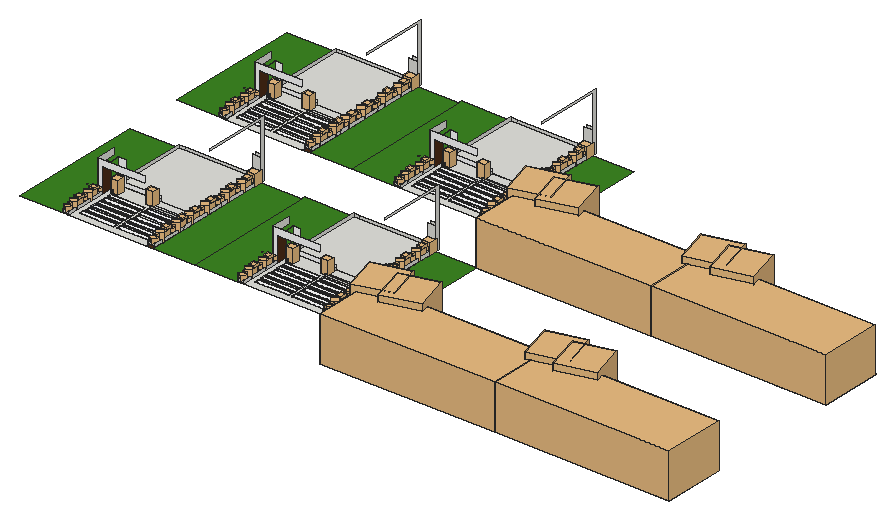
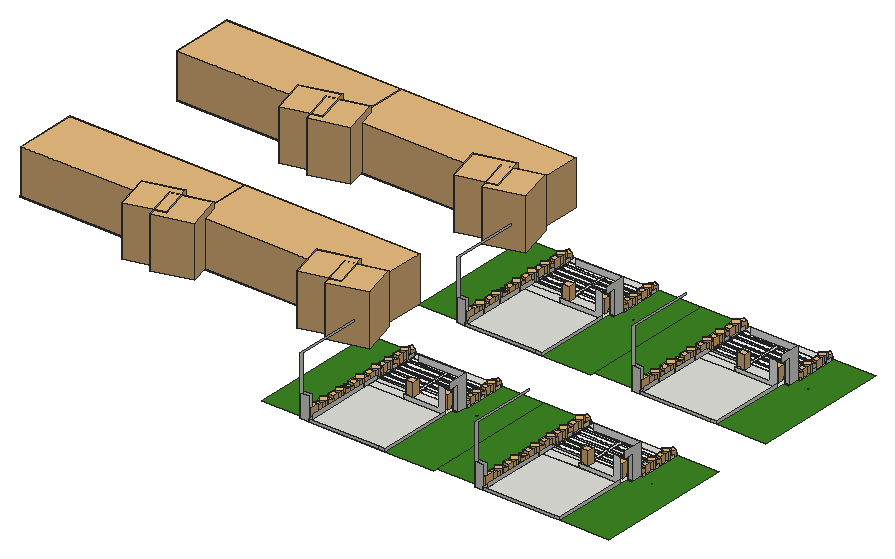
# SketchUp Ruby script. Lengths in inches.
U = 1.inch
M = Sketchup.active_model
def pt(a) = Geom::Point3d.new(a.map { |v| v * U })
def face(e, loops, mat)
  f = e.add_face(loops[0].map { |a| pt(a) })
  loops[1..].each { |l| e.add_face(l.map { |a| pt(a) }).erase! }
  f.material = f.back_material = mat if mat
  f
end
# faces: each face lists its corners as indices into pts; further lists are holes
def faces(e, pts, list, mat = nil) = list.each { |f| face(e, (f[0].is_a?(Array) ? f : [f]).map { |l| l.map { |i| pts[i] } }, mat) }
# xy, xz, yz: faces in a plane at the given z, y or x. An outline is a flat list of corners, or four numbers for a rectangle; further outlines are holes
def ring(l) = l.size == 4 ? [[l[0], l[1]], [l[2], l[1]], [l[2], l[3]], [l[0], l[3]]] : l.each_slice(2).to_a
def flat(e, list, mat, &to3) = list.each { |f| face(e, (f[0].is_a?(Array) ? f : [f]).map { |l| ring(l).map { |u, v| to3.(u, v) } }, mat) }
def xy(e, z, list, mat = nil) = flat(e, list, mat) { |x, y| [x, y, z] }
def xz(e, y, list, mat = nil) = flat(e, list, mat) { |x, z| [x, y, z] }
def yz(e, x, list, mat = nil) = flat(e, list, mat) { |y, z| [x, y, z] }
def lines(e, pts, list) = list.each { |a, b| e.add_line(pt(pts[a]), pt(pts[b])) }
# prism: a flat outline (further loops are holes) pulled along v
def prism(e, loops, v, mat = nil)
  f = face(e, loops, mat); d = Geom::Vector3d.new(v.map { |x| x * U })
  f.pushpull(f.normal.samedirection?(d) ? d.length : -d.length)
end
def box(e, o, s, mat = nil) = prism(e, [[o, [o[0] + s[0], o[1], o[2]], [o[0] + s[0], o[1] + s[1], o[2]], [o[0], o[1] + s[1], o[2]]]], [0, 0, s[2]], mat)
def at(x, y, z, deg = 0) = Geom::Transformation.translation(pt([x, y, z])) * Geom::Transformation.rotation(ORIGIN, Z_AXIS, deg.degrees)
def axes(o, x, y, z) = Geom::Transformation.new([*x, 0, *y, 0, *z, 0, *pt(o).to_a, 1])
def part(name) = M.definitions.add(name)
# library, detail: a bought-in or finely detailed component or shape, given as its bounding box
def library(name, o, s) = part(name).tap { |d| box(d.entities, o, s) }
def detail(e, o, s) = box(e.add_group.entities, o, s)
def put(e, d, t, mat = nil) = e.add_instance(d, t).tap { |i| i.material = mat if mat }
def group(e, t, mat = nil) = e.add_group.tap { |g| g.transformation = t; g.material = mat if mat }.entities
root = M.entities
M.materials.add("Material__1").color = [95, 70, 46]
M.materials.add("[Carrera Marble]").color = [255, 255, 255]
M.materials.add("[Color M00]").color = [255, 255, 255]
M.materials.add("[Color M04]").color = [60, 133, 34]
M.materials.add("[Wood Veneer 01]").color = [76, 44, 23]
c1 = library("plant (1)",[-35.72,-28.42,0],[66.31,67.39,84.38])
c2 = library("Areca palm plant",[0,0,0],[49.1,36.6,54.46])
c3 = library("Group\#14",[-84.69,-90.07,-0.36],[176.51,175.13,171.4])
c4 = library("Group20\#1",[-20.81,-17.08,3.79],[39.86,39.43,37.51])
c5 = library("Group\#130",[-7.34,-1.2,0],[38.67,35.81,49.04])
c6 = library("Group38\#2",[14.01,28.44,-23.43],[18.58,18.32,38.89])
c7 = part("Group\#15")
xy(c7.entities,0,[[0,0,6,234.8],[30,0,36,234.8]])
xy(c7.entities,3,[[6,0,30,234.8]])
xy(c7.entities,7,[[6,5,30,229.8]],"Material__1")
xy(c7.entities,15,[[[0,0,36,234.8],[6,5,30,229.8]]])
xz(c7.entities,0,[[0,0,6,0,6,3,30,3,30,0,36,0,36,15,0,15]])
xz(c7.entities,5,[[6,7,30,15]])
xz(c7.entities,229.8,[[6,7,30,15]])
xz(c7.entities,234.8,[[0,0,0,15,36,15,36,0,30,0,30,3,6,3,6,0]])
yz(c7.entities,0,[[0,0,234.8,15]])
yz(c7.entities,6,[[0,0,234.8,3],[5,7,229.8,15]])
yz(c7.entities,30,[[0,0,234.8,3],[5,7,229.8,15]])
yz(c7.entities,36,[[0,0,234.8,15]])
c8 = part("Group\#17")
put(c8.entities,c2,axes([-6.2,56.6,6.08],[0.45017,-0.56191,0],[0.66137,0.52986,0],[0,0,0.72]))
put(c8.entities,c2,axes([-6.2,158.41,6.08],[0.45017,-0.56191,0],[0.66137,0.52986,0],[0,0,0.72]))
put(c8.entities,c3,axes([14.93,44.05,6.05],[-0.04961,-0.08593,0],[0.08593,-0.04961,0],[0,0,0.10522]))
put(c8.entities,c3,axes([14.93,71.3,6.05],[-0.04961,-0.08593,0],[0.08593,-0.04961,0],[0,0,0.10522]))
put(c8.entities,c4,axes([18.97,79.98,4.77],[0,0.85,0],[-0.85,0,0],[0,0,0.85]))
put(c8.entities,c3,axes([14.93,145.87,6.05],[-0.04961,-0.08593,0],[0.08593,-0.04961,0],[0,0,0.10522]))
put(c8.entities,c3,axes([17.19,15.79,6.07],[-0.08133,-0.14087,0],[0.14087,-0.08133,0],[0,0,0.1725]))
put(c8.entities,c3,axes([17.19,223.04,6.07],[-0.08133,-0.14087,0],[0.14087,-0.08133,0],[0,0,0.1725]))
put(c8.entities,c3,axes([17.19,121.23,6.07],[-0.08133,-0.14087,0],[0.14087,-0.08133,0],[0,0,0.1725]))
put(c8.entities,c5,axes([24.9375,191.72,8],[0,0.79,0],[-0.79,0,0],[0,0,0.79]))
put(c8.entities,c5,axes([24.9375,89.91,8],[0,0.79,0],[-0.79,0,0],[0,0,0.79]))
put(c8.entities,c3,axes([14.93,91.37,6.05],[-0.04961,-0.08593,0],[0.08593,-0.04961,0],[0,0,0.10522]))
put(c8.entities,c4,axes([18.97,181.79,4.77],[0,0.85,0],[-0.85,0,0],[0,0,0.85]))
put(c8.entities,c6,axes([-4.1,-1.15,28.17],[0.8848,0,0],[0,0.94674,0],[0,0,0.85826]))
put(c8.entities,c6,axes([-4.1,100.66,28.17],[0.8848,0,0],[0,0.94674,0],[0,0,0.85826]))
put(c8.entities,c7,at(0,0,0))
put(c8.entities,c3,axes([14.93,173.12,6.05],[-0.04961,-0.08593,0],[0.08593,-0.04961,0],[0,0,0.10522]))
put(c8.entities,c3,axes([14.93,193.18,6.05],[-0.04961,-0.08593,0],[0.08593,-0.04961,0],[0,0,0.10522]))
c9 = library("Plant",[0,0,0],[12.59,12.59,14.16])
c10 = library("plant1",[-367.84,-375.82,-125.45],[750.59,696.16,1346.74])
c11 = part("skp4FF")
put(c11.entities,c10,at(0,0,0))
c12 = library("BPJ-Road5D",[0,0,1],[442,720,229.125])
c13 = library("Palm tree",[-4.09,-4.52,0],[193.52,193.51,258.93])
c14 = part("Palm+Tree")
put(c14.entities,c13,at(25.51,-21.81,0,15))
xy(root,-19.54,[[[279.74,317.81,671.36,317.81,671.36,570.37,491.71,570.37,491.71,638.99,279.74,638.99,279.74,595.43,252.74,595.43,252.74,588.74,279.74,588.74],[493.96,534.6,667.46,556.1],[493.96,464.47,667.46,485.97],[493.96,429.41,667.46,450.91],[493.96,394.35,667.46,415.85],[493.96,359.29,667.46,380.79],[305.46,534.6,478.96,556.1],[305.46,464.47,478.96,485.97],[305.46,429.41,478.96,450.91],[305.46,394.35,478.96,415.85],[305.46,359.29,478.96,380.79],[493.96,499.54,667.46,521.04],[305.46,499.54,478.96,521.04]],[[1172.33,317.81,1563.95,317.81,1563.95,570.37,1384.3,570.37,1384.3,638.99,1172.33,638.99,1172.33,595.43,1145.33,595.43,1145.33,588.74,1172.33,588.74],[1386.55,499.54,1560.05,521.04],[1198.05,499.54,1371.55,521.04],[1386.55,534.6,1560.05,556.1],[1386.55,464.47,1560.05,485.97],[1386.55,429.41,1560.05,450.91],[1386.55,394.35,1560.05,415.85],[1386.55,359.29,1560.05,380.79],[1198.05,534.6,1371.55,556.1],[1198.05,464.47,1371.55,485.97],[1198.05,429.41,1371.55,450.91],[1198.05,394.35,1371.55,415.85],[1198.05,359.29,1371.55,380.79]],[252.74,538.49,279.74,588.74],[1145.33,538.49,1172.33,588.74],[491.71,570.37,671.36,592.87],
  [1384.3,570.37,1563.95,592.87],[491.71,592.87,671.36,638.99],[1384.3,592.87,1563.95,638.99],[279.74,638.99,671.36,1021.31],[1172.33,638.99,1563.95,1021.31],
  [671.36,1001.66,715.11,1021.31],[1563.95,1001.66,1607.7,1021.31],[[279.74,1317.16,671.36,1317.16,671.36,1569.72,491.71,1569.72,491.71,1638.35,279.74,1638.35,279.74,1594.79,252.74,1594.79,252.74,1588.1,279.74,1588.1],[493.96,1533.95,667.46,1555.45],[493.96,1498.89,667.46,1520.39],[493.96,1463.83,667.46,1485.33],[493.96,1428.77,667.46,1450.27],[493.96,1393.7,667.46,1415.2],[493.96,1358.64,667.46,1380.14],[305.46,1533.95,478.96,1555.45],[305.46,1498.89,478.96,1520.39],[305.46,1463.83,478.96,1485.33],[305.46,1428.77,478.96,1450.27],[305.46,1393.7,478.96,1415.2],[305.46,1358.64,478.96,1380.14]],[[1172.33,1317.16,1563.95,1317.16,1563.95,1569.72,1384.3,1569.72,1384.3,1638.35,1172.33,1638.35,1172.33,1594.79,1145.33,1594.79,1145.33,1588.1,1172.33,1588.1],[1386.55,1533.95,1560.05,1555.45],[1386.55,1498.89,1560.05,1520.39],[1386.55,1463.83,1560.05,1485.33],[1386.55,1428.77,1560.05,1450.27],[1386.55,1393.7,1560.05,1415.2],[1386.55,1358.64,1560.05,1380.14],[1198.05,1533.95,1371.55,1555.45],[1198.05,1498.89,1371.55,1520.39],[1198.05,1463.83,1371.55,1485.33],[1198.05,1428.77,1371.55,1450.27],[1198.05,1393.7,1371.55,1415.2],[1198.05,1358.64,1371.55,1380.14]],[252.74,1537.85,279.74,1588.1],
  [1145.33,1537.85,1172.33,1588.1],[491.71,1569.72,671.36,1592.22],[1384.3,1569.72,1563.95,1592.22],[491.71,1592.22,671.36,1638.35],[1384.3,1592.22,1563.95,1638.35],
  [279.74,1638.35,671.36,2020.66],[1172.33,1638.35,1563.95,2020.66],[671.36,2001.02,715.11,2020.66],[1563.95,2001.02,1607.7,2020.66]])
xy(root,-19.54,[[[30.46,317.81,252.74,317.81,252.74,595.43,279.74,595.43,279.74,1021.31,30.46,1021.31],[174.01,564.91,177.17,568.07,177.17,564.91]],[715.11,317.81,923.05,1001.66],[[923.05,317.81,1145.33,317.81,1145.33,595.43,1172.33,595.43,1172.33,1021.31,923.05,1021.31],[1066.6,564.91,1069.76,568.07,1069.76,564.91]],[1607.7,317.81,1815.63,1001.66],[174.01,564.91,177.17,564.91,177.17,568.07],
  [1066.6,564.91,1069.76,564.91,1069.76,568.07],[[30.46,1317.16,252.74,1317.16,252.74,1594.79,279.74,1594.79,279.74,2020.66,30.46,2020.66],[174.01,1564.26,177.17,1567.42,177.17,1564.26]],[715.11,1317.16,923.05,2001.02],[[923.05,1317.16,1145.33,1317.16,1145.33,1594.79,1172.33,1594.79,1172.33,2020.66,923.05,2020.66],[1066.6,1564.26,1069.76,1567.42,1069.76,1564.26]],[1607.7,1317.16,1815.63,2001.02],
  [174.01,1564.26,177.17,1564.26,177.17,1567.42],[1066.6,1564.26,1069.76,1564.26,1069.76,1567.42]],"[Color M04]")
xy(root,-19.54,[[252.74,317.81,279.74,538.49],[671.36,317.81,715.11,1001.66],[1145.33,317.81,1172.33,538.49],[1563.95,317.81,1607.7,1001.66],[252.74,1317.16,279.74,1537.85],
  [671.36,1317.16,715.11,2001.02],[1145.33,1317.16,1172.33,1537.85],[1563.95,1317.16,1607.7,2001.02]],"[Wood Veneer 01]")
xy(root,-18.54,[[1815.63,0,2708.22,315.5],[2708.22,0,3600.8125,315.5],[1815.63,999.35,2708.22,1314.85],[2708.22,999.35,3600.8125,1314.85]])
xy(root,-18.23,[[305.46,359.29,478.96,380.79],[493.96,359.29,667.46,380.79],[1198.05,359.29,1371.55,380.79],[1386.55,359.29,1560.05,380.79],[305.46,394.35,478.96,415.85],
  [493.96,394.35,667.46,415.85],[1198.05,394.35,1371.55,415.85],[1386.55,394.35,1560.05,415.85],[305.46,429.41,478.96,450.91],[493.96,429.41,667.46,450.91],
  [1198.05,429.41,1371.55,450.91],[1386.55,429.41,1560.05,450.91],[305.46,464.47,478.96,485.97],[493.96,464.47,667.46,485.97],[1198.05,464.47,1371.55,485.97],
  [1386.55,464.47,1560.05,485.97],[305.46,499.54,478.96,521.04],[493.96,499.54,667.46,521.04],[1198.05,499.54,1371.55,521.04],[1386.55,499.54,1560.05,521.04],
  [305.46,534.6,478.96,556.1],[493.96,534.6,667.46,556.1],[1198.05,534.6,1371.55,556.1],[1386.55,534.6,1560.05,556.1],[305.46,1358.64,478.96,1380.14],
  [493.96,1358.64,667.46,1380.14],[1198.05,1358.64,1371.55,1380.14],[1386.55,1358.64,1560.05,1380.14],[305.46,1393.7,478.96,1415.2],[493.96,1393.7,667.46,1415.2],
  [1198.05,1393.7,1371.55,1415.2],[1386.55,1393.7,1560.05,1415.2],[305.46,1428.77,478.96,1450.27],[493.96,1428.77,667.46,1450.27],[1198.05,1428.77,1371.55,1450.27],
  [1386.55,1428.77,1560.05,1450.27],[305.46,1463.83,478.96,1485.33],[493.96,1463.83,667.46,1485.33],[1198.05,1463.83,1371.55,1485.33],[1386.55,1463.83,1560.05,1485.33],
  [305.46,1498.89,478.96,1520.39],[493.96,1498.89,667.46,1520.39],[1198.05,1498.89,1371.55,1520.39],[1386.55,1498.89,1560.05,1520.39],[305.46,1533.95,478.96,1555.45],
  [493.96,1533.95,667.46,1555.45],[1198.05,1533.95,1371.55,1555.45],[1386.55,1533.95,1560.05,1555.45]],"[Carrera Marble]")
xz(root,315.5,[[1815.63,-18.54,2708.22,-14.85],[2708.22,-18.54,3600.8125,-14.85]])
xz(root,359.29,[[305.46,-19.54,478.96,-18.23],[493.96,-19.54,667.46,-18.23],[1198.05,-19.54,1371.55,-18.23],[1386.55,-19.54,1560.05,-18.23]])
xz(root,380.79,[[305.46,-19.54,478.96,-18.23],[493.96,-19.54,667.46,-18.23],[1198.05,-19.54,1371.55,-18.23],[1386.55,-19.54,1560.05,-18.23]])
xz(root,394.35,[[305.46,-19.54,478.96,-18.23],[493.96,-19.54,667.46,-18.23],[1198.05,-19.54,1371.55,-18.23],[1386.55,-19.54,1560.05,-18.23]])
xz(root,415.85,[[305.46,-19.54,478.96,-18.23],[493.96,-19.54,667.46,-18.23],[1198.05,-19.54,1371.55,-18.23],[1386.55,-19.54,1560.05,-18.23]])
xz(root,429.41,[[305.46,-19.54,478.96,-18.23],[493.96,-19.54,667.46,-18.23],[1198.05,-19.54,1371.55,-18.23],[1386.55,-19.54,1560.05,-18.23]])
xz(root,450.91,[[305.46,-19.54,478.96,-18.23],[493.96,-19.54,667.46,-18.23],[1198.05,-19.54,1371.55,-18.23],[1386.55,-19.54,1560.05,-18.23]])
xz(root,464.47,[[305.46,-19.54,478.96,-18.23],[493.96,-19.54,667.46,-18.23],[1198.05,-19.54,1371.55,-18.23],[1386.55,-19.54,1560.05,-18.23]])
xz(root,485.97,[[305.46,-19.54,478.96,-18.23],[493.96,-19.54,667.46,-18.23],[1198.05,-19.54,1371.55,-18.23],[1386.55,-19.54,1560.05,-18.23]])
xz(root,499.54,[[305.46,-19.54,478.96,-18.23],[493.96,-19.54,667.46,-18.23],[1198.05,-19.54,1371.55,-18.23],[1386.55,-19.54,1560.05,-18.23]])
xz(root,521.04,[[305.46,-19.54,478.96,-18.23],[493.96,-19.54,667.46,-18.23],[1198.05,-19.54,1371.55,-18.23],[1386.55,-19.54,1560.05,-18.23]])
xz(root,534.6,[[305.46,-19.54,478.96,-18.23],[493.96,-19.54,667.46,-18.23],[1198.05,-19.54,1371.55,-18.23],[1386.55,-19.54,1560.05,-18.23]])
xz(root,538.49,[[252.74,-19.54,279.74,-19.54,279.74,104.9375,491.71,104.9375,491.71,138.1875,252.74,138.1875],[1145.33,-19.54,1172.33,-19.54,1172.33,104.9375,1384.3,104.9375,1384.3,138.1875,1145.33,138.1875]],"[Color M00]")
xz(root,556.1,[[305.46,-19.54,478.96,-18.23],[493.96,-19.54,667.46,-18.23],[1198.05,-19.54,1371.55,-18.23],[1386.55,-19.54,1560.05,-18.23]])
xz(root,570.37,[[491.71,-19.54,671.36,-11.11],[1384.3,-19.54,1563.95,-11.11]])
xz(root,588.74,[[252.74,-19.54,279.74,104.8125],[1145.33,-19.54,1172.33,104.8125]])
xz(root,638.99,[[279.74,-19.54,491.71,-19.54,491.71,1.3125,312.05,1.3125,312.05,104.8125,279.74,104.8125],[1172.33,-19.54,1384.3,-19.54,1384.3,1.3125,1204.64,1.3125,1204.64,104.8125,1172.33,104.8125]],"[Color M00]")
xz(root,999.35,[[2456.54,-18.54,2708.22,-14.85],[3349.13,-18.54,3600.8125,-14.85]])
xz(root,1001.66,[[671.36,-19.54,715.11,97.9375],[1563.95,-19.54,1607.7,97.9375]])
xz(root,1021.31,[[279.74,-19.54,312.05,-4.6875],[312.05,-19.54,671.36,-4.6875],[671.36,-19.54,715.11,97.9375],[1172.33,-19.54,1204.64,-4.6875],[1204.64,-19.54,1563.95,-4.6875],
  [1563.95,-19.54,1607.7,97.9375]])
xz(root,1314.85,[[1815.63,-18.54,2708.22,-14.85],[2708.22,-18.54,3600.8125,-14.85]])
xz(root,1358.64,[[305.46,-19.54,478.96,-18.23],[493.96,-19.54,667.46,-18.23],[1198.05,-19.54,1371.55,-18.23],[1386.55,-19.54,1560.05,-18.23]])
xz(root,1380.14,[[305.46,-19.54,478.96,-18.23],[493.96,-19.54,667.46,-18.23],[1198.05,-19.54,1371.55,-18.23],[1386.55,-19.54,1560.05,-18.23]])
xz(root,1393.7,[[305.46,-19.54,478.96,-18.23],[493.96,-19.54,667.46,-18.23],[1198.05,-19.54,1371.55,-18.23],[1386.55,-19.54,1560.05,-18.23]])
xz(root,1415.2,[[305.46,-19.54,478.96,-18.23],[493.96,-19.54,667.46,-18.23],[1198.05,-19.54,1371.55,-18.23],[1386.55,-19.54,1560.05,-18.23]])
xz(root,1428.77,[[305.46,-19.54,478.96,-18.23],[493.96,-19.54,667.46,-18.23],[1198.05,-19.54,1371.55,-18.23],[1386.55,-19.54,1560.05,-18.23]])
xz(root,1450.27,[[305.46,-19.54,478.96,-18.23],[493.96,-19.54,667.46,-18.23],[1198.05,-19.54,1371.55,-18.23],[1386.55,-19.54,1560.05,-18.23]])
xz(root,1463.83,[[305.46,-19.54,478.96,-18.23],[493.96,-19.54,667.46,-18.23],[1198.05,-19.54,1371.55,-18.23],[1386.55,-19.54,1560.05,-18.23]])
xz(root,1485.33,[[305.46,-19.54,478.96,-18.23],[493.96,-19.54,667.46,-18.23],[1198.05,-19.54,1371.55,-18.23],[1386.55,-19.54,1560.05,-18.23]])
xz(root,1498.89,[[305.46,-19.54,478.96,-18.23],[493.96,-19.54,667.46,-18.23],[1198.05,-19.54,1371.55,-18.23],[1386.55,-19.54,1560.05,-18.23]])
xz(root,1520.39,[[305.46,-19.54,478.96,-18.23],[493.96,-19.54,667.46,-18.23],[1198.05,-19.54,1371.55,-18.23],[1386.55,-19.54,1560.05,-18.23]])
xz(root,1533.95,[[305.46,-19.54,478.96,-18.23],[493.96,-19.54,667.46,-18.23],[1198.05,-19.54,1371.55,-18.23],[1386.55,-19.54,1560.05,-18.23]])
xz(root,1537.85,[[252.74,-19.54,279.74,-19.54,279.74,104.9375,491.71,104.9375,491.71,138.1875,252.74,138.1875],[1145.33,-19.54,1172.33,-19.54,1172.33,104.9375,1384.3,104.9375,1384.3,138.1875,1145.33,138.1875]],"[Color M00]")
xz(root,1555.45,[[305.46,-19.54,478.96,-18.23],[493.96,-19.54,667.46,-18.23],[1198.05,-19.54,1371.55,-18.23],[1386.55,-19.54,1560.05,-18.23]])
xz(root,1569.72,[[491.71,-19.54,671.36,-11.11],[1384.3,-19.54,1563.95,-11.11]])
xz(root,1588.1,[[252.74,-19.54,279.74,104.8125],[1145.33,-19.54,1172.33,104.8125]])
xz(root,1638.35,[[279.74,-19.54,491.71,-19.54,491.71,1.3125,312.05,1.3125,312.05,104.8125,279.74,104.8125],[1172.33,-19.54,1384.3,-19.54,1384.3,1.3125,1204.64,1.3125,1204.64,104.8125,1172.33,104.8125]],"[Color M00]")
xz(root,2001.02,[[671.36,-19.54,715.11,97.9375],[1563.95,-19.54,1607.7,97.9375]])
xz(root,2020.66,[[279.74,-19.54,312.05,-4.6875],[312.05,-19.54,671.36,-4.6875],[671.36,-19.54,715.11,97.9375],[1172.33,-19.54,1204.64,-4.6875],[1204.64,-19.54,1563.95,-4.6875],
  [1563.95,-19.54,1607.7,97.9375]])
yz(root,252.74,[[538.49,-19.54,538.49,138.1875,638.99,138.1875,638.99,104.8125,588.74,104.8125,588.74,-19.54],[1537.85,-19.54,1537.85,138.1875,1638.35,138.1875,1638.35,104.8125,1588.1,104.8125,1588.1,-19.54]])
yz(root,279.74,[[638.99,-19.54,1021.31,-4.6875],[1638.35,-19.54,2020.66,-4.6875]])
yz(root,279.74,[[538.49,-19.54,588.74,-19.54,588.74,104.8125,638.99,104.8125,638.99,104.9375,538.49,104.9375],[1537.85,-19.54,1588.1,-19.54,1588.1,104.8125,1638.35,104.8125,1638.35,104.9375,1537.85,104.9375]],"[Wood Veneer 01]")
yz(root,305.46,[[359.29,-19.54,380.79,-18.23],[394.35,-19.54,415.85,-18.23],[429.41,-19.54,450.91,-18.23],[464.47,-19.54,485.97,-18.23],[499.54,-19.54,521.04,-18.23],
  [534.6,-19.54,556.1,-18.23],[1358.64,-19.54,1380.14,-18.23],[1393.7,-19.54,1415.2,-18.23],[1428.77,-19.54,1450.27,-18.23],[1463.83,-19.54,1485.33,-18.23],
  [1498.89,-19.54,1520.39,-18.23],[1533.95,-19.54,1555.45,-18.23]])
yz(root,478.96,[[359.29,-19.54,380.79,-18.23],[394.35,-19.54,415.85,-18.23],[429.41,-19.54,450.91,-18.23],[464.47,-19.54,485.97,-18.23],[499.54,-19.54,521.04,-18.23],
  [534.6,-19.54,556.1,-18.23],[1358.64,-19.54,1380.14,-18.23],[1393.7,-19.54,1415.2,-18.23],[1428.77,-19.54,1450.27,-18.23],[1463.83,-19.54,1485.33,-18.23],
  [1498.89,-19.54,1520.39,-18.23],[1533.95,-19.54,1555.45,-18.23]])
yz(root,491.71,[[570.37,-19.54,592.87,-11.11],[592.87,-19.54,638.99,-11.11],[1569.72,-19.54,1592.22,-11.11],[1592.22,-19.54,1638.35,-11.11]])
yz(root,493.96,[[359.29,-19.54,380.79,-18.23],[394.35,-19.54,415.85,-18.23],[429.41,-19.54,450.91,-18.23],[464.47,-19.54,485.97,-18.23],[499.54,-19.54,521.04,-18.23],
  [534.6,-19.54,556.1,-18.23],[1358.64,-19.54,1380.14,-18.23],[1393.7,-19.54,1415.2,-18.23],[1428.77,-19.54,1450.27,-18.23],[1463.83,-19.54,1485.33,-18.23],
  [1498.89,-19.54,1520.39,-18.23],[1533.95,-19.54,1555.45,-18.23]])
yz(root,667.46,[[359.29,-19.54,380.79,-18.23],[394.35,-19.54,415.85,-18.23],[429.41,-19.54,450.91,-18.23],[464.47,-19.54,485.97,-18.23],[499.54,-19.54,521.04,-18.23],
  [534.6,-19.54,556.1,-18.23],[1358.64,-19.54,1380.14,-18.23],[1393.7,-19.54,1415.2,-18.23],[1428.77,-19.54,1450.27,-18.23],[1463.83,-19.54,1485.33,-18.23],
  [1498.89,-19.54,1520.39,-18.23],[1533.95,-19.54,1555.45,-18.23]])
yz(root,671.36,[[570.37,-19.54,1001.66,-19.54,1001.66,1.3125,592.87,1.3125,592.87,-4.74,582.24,-4.74,582.24,-11.11,570.37,-11.11],[1001.66,-19.54,1021.31,-4.6875],[1569.72,-19.54,2001.02,-19.54,2001.02,1.3125,1592.22,1.3125,1592.22,-4.74,1581.6,-4.74,1581.6,-11.11,1569.72,-11.11],[2001.02,-19.54,2020.66,-4.6875]])
yz(root,715.11,[[1001.66,-19.54,1021.31,-19.54,1021.31,279.25,676.67,279.25,676.67,269.375,1001.66,269.375],[2001.02,-19.54,2020.66,-19.54,2020.66,279.25,1676.03,279.25,1676.03,269.375,2001.02,269.375]])
yz(root,1145.33,[[538.49,-19.54,538.49,138.1875,638.99,138.1875,638.99,104.8125,588.74,104.8125,588.74,-19.54],[1537.85,-19.54,1537.85,138.1875,1638.35,138.1875,1638.35,104.8125,1588.1,104.8125,1588.1,-19.54]])
yz(root,1172.33,[[638.99,-19.54,1021.31,-4.6875],[1638.35,-19.54,2020.66,-4.6875]])
yz(root,1172.33,[[538.49,-19.54,588.74,-19.54,588.74,104.8125,638.99,104.8125,638.99,104.9375,538.49,104.9375],[1537.85,-19.54,1588.1,-19.54,1588.1,104.8125,1638.35,104.8125,1638.35,104.9375,1537.85,104.9375]],"[Wood Veneer 01]")
yz(root,1198.05,[[359.29,-19.54,380.79,-18.23],[394.35,-19.54,415.85,-18.23],[429.41,-19.54,450.91,-18.23],[464.47,-19.54,485.97,-18.23],[499.54,-19.54,521.04,-18.23],
  [534.6,-19.54,556.1,-18.23],[1358.64,-19.54,1380.14,-18.23],[1393.7,-19.54,1415.2,-18.23],[1428.77,-19.54,1450.27,-18.23],[1463.83,-19.54,1485.33,-18.23],
  [1498.89,-19.54,1520.39,-18.23],[1533.95,-19.54,1555.45,-18.23]])
yz(root,1371.55,[[359.29,-19.54,380.79,-18.23],[394.35,-19.54,415.85,-18.23],[429.41,-19.54,450.91,-18.23],[464.47,-19.54,485.97,-18.23],[499.54,-19.54,521.04,-18.23],
  [534.6,-19.54,556.1,-18.23],[1358.64,-19.54,1380.14,-18.23],[1393.7,-19.54,1415.2,-18.23],[1428.77,-19.54,1450.27,-18.23],[1463.83,-19.54,1485.33,-18.23],
  [1498.89,-19.54,1520.39,-18.23],[1533.95,-19.54,1555.45,-18.23]])
yz(root,1384.3,[[570.37,-19.54,592.87,-11.11],[592.87,-19.54,638.99,-11.11],[1569.72,-19.54,1592.22,-11.11],[1592.22,-19.54,1638.35,-11.11]])
yz(root,1386.55,[[359.29,-19.54,380.79,-18.23],[394.35,-19.54,415.85,-18.23],[429.41,-19.54,450.91,-18.23],[464.47,-19.54,485.97,-18.23],[499.54,-19.54,521.04,-18.23],
  [534.6,-19.54,556.1,-18.23],[1358.64,-19.54,1380.14,-18.23],[1393.7,-19.54,1415.2,-18.23],[1428.77,-19.54,1450.27,-18.23],[1463.83,-19.54,1485.33,-18.23],
  [1498.89,-19.54,1520.39,-18.23],[1533.95,-19.54,1555.45,-18.23]])
yz(root,1560.05,[[359.29,-19.54,380.79,-18.23],[394.35,-19.54,415.85,-18.23],[429.41,-19.54,450.91,-18.23],[464.47,-19.54,485.97,-18.23],[499.54,-19.54,521.04,-18.23],
  [534.6,-19.54,556.1,-18.23],[1358.64,-19.54,1380.14,-18.23],[1393.7,-19.54,1415.2,-18.23],[1428.77,-19.54,1450.27,-18.23],[1463.83,-19.54,1485.33,-18.23],
  [1498.89,-19.54,1520.39,-18.23],[1533.95,-19.54,1555.45,-18.23]])
yz(root,1563.95,[[570.37,-19.54,1001.66,-19.54,1001.66,1.3125,592.87,1.3125,592.87,-4.74,582.24,-4.74,582.24,-11.11,570.37,-11.11],[1001.66,-19.54,1021.31,-4.6875],[1569.72,-19.54,2001.02,-19.54,2001.02,1.3125,1592.22,1.3125,1592.22,-4.74,1581.6,-4.74,1581.6,-11.11,1569.72,-11.11],[2001.02,-19.54,2020.66,-4.6875]])
yz(root,1607.7,[[1001.66,-19.54,1021.31,-19.54,1021.31,279.25,676.67,279.25,676.67,269.375,1001.66,269.375],[2001.02,-19.54,2020.66,-19.54,2020.66,279.25,1676.03,279.25,1676.03,269.375,2001.02,269.375]])
yz(root,2708.22,[[999.35,-18.54,1019,-14.85]])
put(root,c1,axes([695.3,1980.36,-19.54],[0.67,0,0],[0,0.67,0],[0,0,0.67]))
put(root,c8,at(675,1513.78,-19.54))
put(root,c8,at(675,1744.41,-19.54))
put(root,c1,axes([695.3,981,-19.54],[0.67,0,0],[0,0.67,0],[0,0,0.67]))
put(root,c8,at(675,514.43,-19.54))
put(root,c8,at(675,745.05,-19.54))
put(root,c8,at(675,1329.83,-19.54))
put(root,c8,at(675,330.48,-19.54))
put(root,c8,axes([244.94,1320.89,-19.54],[0.92,0,0],[0,0.92,0],[0,0,0.92]))
put(root,c8,axes([244.94,321.54,-19.54],[0.92,0,0],[0,0.92,0],[0,0,0.92]))
put(root,c1,axes([1587.89,1980.36,-19.54],[0.67,0,0],[0,0.67,0],[0,0,0.67]))
put(root,c8,at(1567.59,1513.78,-19.54))
put(root,c8,at(1567.59,1744.41,-19.54))
put(root,c1,axes([1587.89,981,-19.54],[0.67,0,0],[0,0.67,0],[0,0,0.67]))
put(root,c8,at(1567.59,514.43,-19.54))
put(root,c8,at(1567.59,745.05,-19.54))
put(root,c8,at(1567.59,1329.83,-19.54))
put(root,c8,at(1567.59,330.48,-19.54))
put(root,c8,axes([1137.53,1320.89,-19.54],[0.92,0,0],[0,0.92,0],[0,0,0.92]))
put(root,c8,axes([1137.53,321.54,-19.54],[0.92,0,0],[0,0.92,0],[0,0,0.92]))
put(root,c9,at(295.05,1565.41,-18.23))
put(root,c11,axes([314.32,1585.11,-11.89],[0.05049,0,0],[0,0.05049,0],[0,0,0.05049]))
put(root,c9,at(295.05,566.05,-18.23))
put(root,c11,axes([314.32,585.75,-11.89],[0.05049,0,0],[0,0.05049,0],[0,0,0.05049]))
put(root,c9,at(1187.64,1565.41,-18.23))
put(root,c11,axes([1206.91,1585.11,-11.89],[0.05049,0,0],[0,0.05049,0],[0,0,0.05049]))
put(root,c9,at(1187.64,566.05,-18.23))
put(root,c11,axes([1206.91,585.75,-11.89],[0.05049,0,0],[0,0.05049,0],[0,0,0.05049]))
put(root,c12,axes([2708.22,997.05,-18.54],[0,0.71,0],[-1.23971,0,0],[0,0,1]))
put(root,c12,axes([2708.22,-2.31,-18.54],[0,0.71,0],[-1.23971,0,0],[0,0,1]))
put(root,c12,axes([3600.8125,997.05,-18.54],[0,0.71,0],[-1.23971,0,0],[0,0,1]))
put(root,c12,axes([3600.8125,-2.31,-18.54],[0,0.71,0],[-1.23971,0,0],[0,0,1]))
put(root,c14,at(1768.43,1250.14,-17.51))
put(root,c14,at(1768.43,250.79,-17.51))
put(root,c14,at(2661.02,1250.14,-17.51))
put(root,c14,at(2661.02,250.79,-17.51))
put(root,c11,axes([483.67,1594.61,-10.61],[0.05049,0,0],[0,0.05049,0],[0,0,0.05049]))
put(root,c11,axes([483.67,595.25,-10.61],[0.05049,0,0],[0,0.05049,0],[0,0,0.05049]))
put(root,c11,axes([1376.25,1594.61,-10.61],[0.05049,0,0],[0,0.05049,0],[0,0,0.05049]))
put(root,c11,axes([1376.25,595.25,-10.61],[0.05049,0,0],[0,0.05049,0],[0,0,0.05049]))
put(root,c14,at(1913.02,1248.11,-16.2))
put(root,c14,at(1913.02,248.75,-16.2))
put(root,c14,at(2805.61,1248.11,-16.2))
put(root,c14,at(2805.61,248.75,-16.2))
